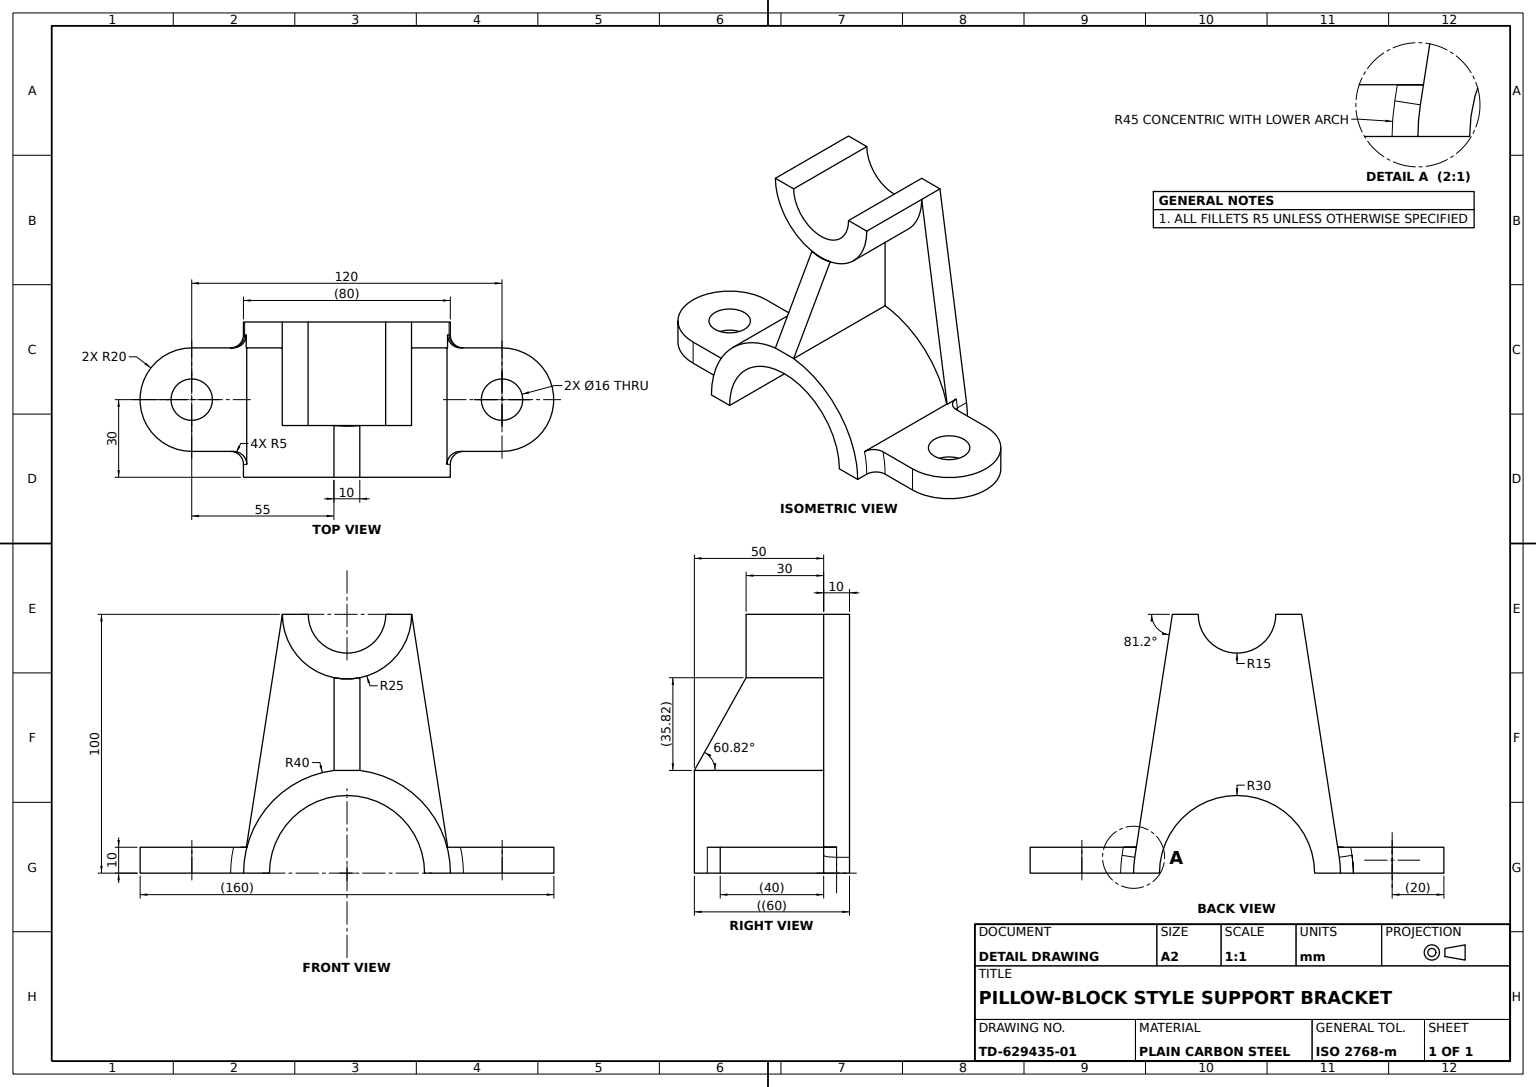
ISO-10303-21;
HEADER;
FILE_DESCRIPTION((''),'2;1');
FILE_NAME('','',(''),(''),'','','');
FILE_SCHEMA(('AUTOMOTIVE_DESIGN'));
ENDSEC;
DATA;
#1=APPLICATION_CONTEXT('');
#2=PRODUCT_CONTEXT('',#1,'mechanical');
#3=PRODUCT('','','',(#2));
#4=PRODUCT_DEFINITION_FORMATION('','',#3);
#5=PRODUCT_DEFINITION_CONTEXT('',#1,'design');
#6=PRODUCT_DEFINITION('','',#4,#5);
#7=PRODUCT_DEFINITION_SHAPE('','',#6);
#8=(LENGTH_UNIT()NAMED_UNIT(*)SI_UNIT(.MILLI.,.METRE.));
#9=(NAMED_UNIT(*)PLANE_ANGLE_UNIT()SI_UNIT($,.RADIAN.));
#10=(NAMED_UNIT(*)SI_UNIT($,.STERADIAN.)SOLID_ANGLE_UNIT());
#11=UNCERTAINTY_MEASURE_WITH_UNIT(LENGTH_MEASURE(1.E-05),#8,'distance_accuracy_value','');
#12=(GEOMETRIC_REPRESENTATION_CONTEXT(3)GLOBAL_UNCERTAINTY_ASSIGNED_CONTEXT((#11))GLOBAL_UNIT_ASSIGNED_CONTEXT((#8,#9,#10))REPRESENTATION_CONTEXT('',''));
#13=CARTESIAN_POINT('',(60.,0.,10.));
#14=VERTEX_POINT('',#13);
#15=CARTESIAN_POINT('',(60.,0.,50.));
#16=VERTEX_POINT('',#15);
#17=CARTESIAN_POINT('',(60.,0.,30.));
#18=DIRECTION('',(0.,-1.,0.));
#19=DIRECTION('',(0.,0.,-1.));
#20=AXIS2_PLACEMENT_3D('',#17,#18,#19);
#21=CIRCLE('',#20,20.);
#22=EDGE_CURVE('',#14,#16,#21,.T.);
#23=ORIENTED_EDGE('',*,*,#22,.T.);
#24=CARTESIAN_POINT('',(45.,0.,50.));
#25=VERTEX_POINT('',#24);
#26=DIRECTION('',(-1.,0.,0.));
#27=VECTOR('',#26,1000.);
#28=LINE('',#15,#27);
#29=EDGE_CURVE('',#16,#25,#28,.T.);
#30=ORIENTED_EDGE('',*,*,#29,.T.);
#31=CARTESIAN_POINT('',(40.,0.,55.));
#32=VERTEX_POINT('',#31);
#33=CARTESIAN_POINT('',(45.,0.,55.));
#34=DIRECTION('',(0.,1.,0.));
#35=DIRECTION('',(0.,0.,1.));
#36=AXIS2_PLACEMENT_3D('',#33,#34,#35);
#37=CIRCLE('',#36,5.);
#38=EDGE_CURVE('',#25,#32,#37,.T.);
#39=ORIENTED_EDGE('',*,*,#38,.T.);
#40=CARTESIAN_POINT('',(40.,0.,60.));
#41=VERTEX_POINT('',#40);
#42=CARTESIAN_POINT('',(40.,0.,50.));
#43=VECTOR('',#19,1000.);
#44=LINE('',#42,#43);
#45=EDGE_CURVE('',#41,#32,#44,.T.);
#46=ORIENTED_EDGE('',*,*,#45,.F.);
#47=CARTESIAN_POINT('',(30.,0.,60.));
#48=VERTEX_POINT('',#47);
#49=DIRECTION('',(1.,0.,0.));
#50=VECTOR('',#49,1000.);
#51=LINE('',#47,#50);
#52=EDGE_CURVE('',#48,#41,#51,.T.);
#53=ORIENTED_EDGE('',*,*,#52,.F.);
#54=CARTESIAN_POINT('',(30.,0.,0.));
#55=VERTEX_POINT('',#54);
#56=CARTESIAN_POINT('',(30.,0.,50.));
#57=LINE('',#56,#43);
#58=EDGE_CURVE('',#48,#55,#57,.T.);
#59=ORIENTED_EDGE('',*,*,#58,.T.);
#60=CARTESIAN_POINT('',(40.,0.,0.));
#61=VERTEX_POINT('',#60);
#62=LINE('',#54,#50);
#63=EDGE_CURVE('',#55,#61,#62,.T.);
#64=ORIENTED_EDGE('',*,*,#63,.T.);
#65=CARTESIAN_POINT('',(40.,0.,5.));
#66=VERTEX_POINT('',#65);
#67=EDGE_CURVE('',#66,#61,#44,.T.);
#68=ORIENTED_EDGE('',*,*,#67,.F.);
#69=CARTESIAN_POINT('',(45.,0.,10.));
#70=VERTEX_POINT('',#69);
#71=CARTESIAN_POINT('',(45.,0.,5.));
#72=AXIS2_PLACEMENT_3D('',#71,#34,#35);
#73=CIRCLE('',#72,5.);
#74=EDGE_CURVE('',#66,#70,#73,.T.);
#75=ORIENTED_EDGE('',*,*,#74,.T.);
#76=LINE('',#13,#50);
#77=EDGE_CURVE('',#70,#14,#76,.T.);
#78=ORIENTED_EDGE('',*,*,#77,.T.);
#79=EDGE_LOOP('',(#23,#30,#39,#46,#53,#59,#64,#68,#75,#78));
#80=FACE_OUTER_BOUND('',#79,.T.);
#81=CARTESIAN_POINT('',(60.,0.,22.));
#82=VERTEX_POINT('',#81);
#83=CARTESIAN_POINT('',(60.,0.,38.));
#84=VERTEX_POINT('',#83);
#85=CIRCLE('',#20,8.);
#86=EDGE_CURVE('',#82,#84,#85,.T.);
#87=ORIENTED_EDGE('',*,*,#86,.F.);
#88=EDGE_CURVE('',#84,#82,#85,.T.);
#89=ORIENTED_EDGE('',*,*,#88,.F.);
#90=EDGE_LOOP('',(#87,#89));
#91=FACE_BOUND('',#90,.T.);
#92=AXIS2_PLACEMENT_3D('',#56,#34,#35);
#93=PLANE('',#92);
#94=ADVANCED_FACE('',(#80,#91),#93,.F.);
#95=CARTESIAN_POINT('',(5.,75.505103,20.));
#96=VERTEX_POINT('',#95);
#97=CARTESIAN_POINT('',(-5.,75.505103,20.));
#98=VERTEX_POINT('',#97);
#99=CARTESIAN_POINT('',(1.689422,74.829334,19.622674));
#100=CARTESIAN_POINT('',(-1.689422,74.829334,19.622674));
#101=(BOUNDED_CURVE()B_SPLINE_CURVE(3,(#95,#99,#100,#97),.UNSPECIFIED.,.F.,.F.)B_SPLINE_CURVE_WITH_KNOTS((4,4),(2.940234733,3.342950574),.UNSPECIFIED.)CURVE()GEOMETRIC_REPRESENTATION_ITEM()RATIONAL_B_SPLINE_CURVE((1.,0.986530598,0.986530598,1.))REPRESENTATION_ITEM(''));
#102=EDGE_CURVE('',#96,#98,#101,.T.);
#103=ORIENTED_EDGE('',*,*,#102,.F.);
#104=CARTESIAN_POINT('',(5.,39.68627,0.));
#105=VERTEX_POINT('',#104);
#106=CARTESIAN_POINT('',(5.,51.162369,6.407858));
#107=DIRECTION('',(0.,0.873113733,0.487516573));
#108=VECTOR('',#107,1000.);
#109=LINE('',#106,#108);
#110=EDGE_CURVE('',#105,#96,#109,.T.);
#111=ORIENTED_EDGE('',*,*,#110,.F.);
#112=CARTESIAN_POINT('',(-5.,39.68627,0.));
#113=VERTEX_POINT('',#112);
#114=CARTESIAN_POINT('',(10.,39.68627,0.));
#115=LINE('',#114,#27);
#116=EDGE_CURVE('',#105,#113,#115,.T.);
#117=ORIENTED_EDGE('',*,*,#116,.T.);
#118=LINE('',#97,#108);
#119=EDGE_CURVE('',#113,#98,#118,.T.);
#120=ORIENTED_EDGE('',*,*,#119,.T.);
#121=EDGE_LOOP('',(#103,#111,#117,#120));
#122=FACE_OUTER_BOUND('',#121,.T.);
#123=CARTESIAN_POINT('',(10.,75.505103,20.));
#124=DIRECTION('',(0.,-0.487516573,0.873113733));
#125=DIRECTION('',(0.,-0.873113733,-0.487516573));
#126=AXIS2_PLACEMENT_3D('',#123,#124,#125);
#127=PLANE('',#126);
#128=ADVANCED_FACE('',(#122),#127,.F.);
#129=CARTESIAN_POINT('',(5.,39.68627,50.));
#130=VERTEX_POINT('',#129);
#131=CARTESIAN_POINT('',(38.729833,10.,50.));
#132=VERTEX_POINT('',#131);
#133=CARTESIAN_POINT('',(0.,0.,50.));
#134=AXIS2_PLACEMENT_3D('',#133,#19,#49);
#135=CIRCLE('',#134,40.);
#136=EDGE_CURVE('',#130,#132,#135,.T.);
#137=ORIENTED_EDGE('',*,*,#136,.T.);
#138=CARTESIAN_POINT('',(38.729833,10.,5.));
#139=VERTEX_POINT('',#138);
#140=VECTOR('',#35,1000.);
#141=LINE('',#131,#140);
#142=EDGE_CURVE('',#139,#132,#141,.T.);
#143=ORIENTED_EDGE('',*,*,#142,.F.);
#144=CARTESIAN_POINT('',(0.,0.,5.));
#145=AXIS2_PLACEMENT_3D('',#144,#19,#49);
#146=CIRCLE('',#145,40.);
#147=EDGE_CURVE('',#139,#66,#146,.T.);
#148=ORIENTED_EDGE('',*,*,#147,.T.);
#149=ORIENTED_EDGE('',*,*,#67,.T.);
#150=CARTESIAN_POINT('',(0.,0.,0.));
#151=AXIS2_PLACEMENT_3D('',#150,#35,#49);
#152=CIRCLE('',#151,40.);
#153=EDGE_CURVE('',#61,#105,#152,.T.);
#154=ORIENTED_EDGE('',*,*,#153,.T.);
#155=CARTESIAN_POINT('',(5.,39.68627,-37.188557));
#156=LINE('',#155,#140);
#157=EDGE_CURVE('',#105,#130,#156,.T.);
#158=ORIENTED_EDGE('',*,*,#157,.T.);
#159=EDGE_LOOP('',(#137,#143,#148,#149,#154,#158));
#160=FACE_OUTER_BOUND('',#159,.T.);
#161=AXIS2_PLACEMENT_3D('',#133,#19,#26);
#162=CYLINDRICAL_SURFACE('',#161,40.);
#163=ADVANCED_FACE('',(#160),#162,.T.);
#164=ORIENTED_EDGE('',*,*,#77,.F.);
#165=CARTESIAN_POINT('',(43.874822,10.,10.));
#166=VERTEX_POINT('',#165);
#167=CARTESIAN_POINT('',(0.,0.,10.));
#168=AXIS2_PLACEMENT_3D('',#167,#35,#49);
#169=CIRCLE('',#168,45.);
#170=EDGE_CURVE('',#70,#166,#169,.T.);
#171=ORIENTED_EDGE('',*,*,#170,.T.);
#172=CARTESIAN_POINT('',(60.,10.,10.));
#173=VERTEX_POINT('',#172);
#174=CARTESIAN_POINT('',(35.,10.,10.));
#175=LINE('',#174,#50);
#176=EDGE_CURVE('',#166,#173,#175,.T.);
#177=ORIENTED_EDGE('',*,*,#176,.T.);
#178=VECTOR('',#18,1000.);
#179=LINE('',#172,#178);
#180=EDGE_CURVE('',#173,#14,#179,.T.);
#181=ORIENTED_EDGE('',*,*,#180,.T.);
#182=EDGE_LOOP('',(#164,#171,#177,#181));
#183=FACE_OUTER_BOUND('',#182,.T.);
#184=AXIS2_PLACEMENT_3D('',#174,#35,#49);
#185=PLANE('',#184);
#186=ADVANCED_FACE('',(#183),#185,.F.);
#187=ORIENTED_EDGE('',*,*,#157,.F.);
#188=ORIENTED_EDGE('',*,*,#110,.T.);
#189=CARTESIAN_POINT('',(5.,75.505103,50.));
#190=VERTEX_POINT('',#189);
#191=CARTESIAN_POINT('',(5.,75.505103,-37.188557));
#192=LINE('',#191,#140);
#193=EDGE_CURVE('',#96,#190,#192,.T.);
#194=ORIENTED_EDGE('',*,*,#193,.T.);
#195=LINE('',#189,#178);
#196=EDGE_CURVE('',#190,#130,#195,.T.);
#197=ORIENTED_EDGE('',*,*,#196,.T.);
#198=EDGE_LOOP('',(#187,#188,#194,#197));
#199=FACE_OUTER_BOUND('',#198,.T.);
#200=AXIS2_PLACEMENT_3D('',#191,#26,#35);
#201=PLANE('',#200);
#202=ADVANCED_FACE('',(#199),#201,.F.);
#203=CARTESIAN_POINT('',(-43.874822,10.,10.));
#204=VERTEX_POINT('',#203);
#205=CARTESIAN_POINT('',(-45.,0.,10.));
#206=VERTEX_POINT('',#205);
#207=EDGE_CURVE('',#204,#206,#169,.T.);
#208=ORIENTED_EDGE('',*,*,#207,.F.);
#209=CARTESIAN_POINT('',(-38.729833,10.,5.));
#210=VERTEX_POINT('',#209);
#211=CARTESIAN_POINT('',(-38.729833,10.,5.334921));
#212=CARTESIAN_POINT('',(-38.764239,10.,5.663939));
#213=CARTESIAN_POINT('',(-38.898767,10.,6.310699));
#214=CARTESIAN_POINT('',(-39.000686,10.,6.631925));
#215=CARTESIAN_POINT('',(-39.26464,10.,7.240754));
#216=CARTESIAN_POINT('',(-39.425819,10.,7.528988));
#217=CARTESIAN_POINT('',(-39.805716,10.,8.073571));
#218=CARTESIAN_POINT('',(-40.024896,10.,8.328981));
#219=CARTESIAN_POINT('',(-40.501992,10.,8.786245));
#220=CARTESIAN_POINT('',(-40.762043,10.,8.99135));
#221=CARTESIAN_POINT('',(-41.325287,10.,9.352802));
#222=CARTESIAN_POINT('',(-41.619798,10.,9.503625));
#223=CARTESIAN_POINT('',(-42.233333,10.,9.748401));
#224=CARTESIAN_POINT('',(-42.555336,10.,9.842795));
#225=CARTESIAN_POINT('',(-43.209353,10.,9.968362));
#226=CARTESIAN_POINT('',(-43.540159,10.,10.));
#227=B_SPLINE_CURVE_WITH_KNOTS('',3,(#209,#211,#212,#213,#214,#215,#216,#217,#218,#219,#220,#221,#222,#223,#224,#225,#226,#203),.UNSPECIFIED.,.F.,.F.,(4,2,2,2,2,2,2,2,4),(0.,0.000990292,0.001980584,0.002970876,0.003961168,0.00495146,0.005941752,0.006932044,0.007922336),.UNSPECIFIED.);
#228=EDGE_CURVE('',#210,#204,#227,.T.);
#229=ORIENTED_EDGE('',*,*,#228,.F.);
#230=CARTESIAN_POINT('',(-40.,0.,5.));
#231=VERTEX_POINT('',#230);
#232=EDGE_CURVE('',#231,#210,#146,.T.);
#233=ORIENTED_EDGE('',*,*,#232,.F.);
#234=CARTESIAN_POINT('',(-45.,0.,5.));
#235=AXIS2_PLACEMENT_3D('',#234,#34,#35);
#236=CIRCLE('',#235,5.);
#237=EDGE_CURVE('',#206,#231,#236,.T.);
#238=ORIENTED_EDGE('',*,*,#237,.F.);
#239=EDGE_LOOP('',(#208,#229,#233,#238));
#240=FACE_OUTER_BOUND('',#239,.T.);
#241=AXIS2_PLACEMENT_3D('',#144,#35,#49);
#242=TOROIDAL_SURFACE('',#241,45.,5.);
#243=ADVANCED_FACE('',(#240),#242,.F.);
#244=ORIENTED_EDGE('',*,*,#147,.F.);
#245=CARTESIAN_POINT('',(43.539992,10.,10.));
#246=CARTESIAN_POINT('',(43.21054,10.,9.968335));
#247=CARTESIAN_POINT('',(42.724094,10.,9.875321));
#248=CARTESIAN_POINT('',(42.563243,10.,9.836674));
#249=CARTESIAN_POINT('',(42.244192,10.,9.743772));
#250=CARTESIAN_POINT('',(42.085245,10.,9.689167));
#251=CARTESIAN_POINT('',(41.621523,10.,9.504613));
#252=CARTESIAN_POINT('',(41.327745,10.,9.353874));
#253=CARTESIAN_POINT('',(40.770701,10.,8.997402));
#254=CARTESIAN_POINT('',(40.505176,10.,8.788985));
#255=CARTESIAN_POINT('',(40.026677,10.,8.330996));
#256=CARTESIAN_POINT('',(39.811545,10.,8.080827));
#257=CARTESIAN_POINT('',(39.525925,10.,7.673018));
#258=CARTESIAN_POINT('',(39.436488,10.,7.530735));
#259=CARTESIAN_POINT('',(39.273687,10.,7.240064));
#260=CARTESIAN_POINT('',(39.200154,10.,7.091651));
#261=CARTESIAN_POINT('',(39.002728,10.,6.637342));
#262=CARTESIAN_POINT('',(38.901772,10.,6.322474));
#263=CARTESIAN_POINT('',(38.764431,10.,5.667473));
#264=CARTESIAN_POINT('',(38.729833,10.,5.335102));
#265=B_SPLINE_CURVE_WITH_KNOTS('',3,(#165,#245,#246,#247,#248,#249,#250,#251,#252,#253,#254,#255,#256,#257,#258,#259,#260,#261,#262,#263,#264,#138),.UNSPECIFIED.,.F.,.F.,(4,2,2,2,2,2,2,2,2,2,4),(0.,0.000990307,0.001485461,0.001980615,0.002970922,0.003961229,0.004951537,0.00544669,0.005941844,0.006932151,0.007922459),.UNSPECIFIED.);
#266=EDGE_CURVE('',#166,#139,#265,.T.);
#267=ORIENTED_EDGE('',*,*,#266,.F.);
#268=ORIENTED_EDGE('',*,*,#170,.F.);
#269=ORIENTED_EDGE('',*,*,#74,.F.);
#270=EDGE_LOOP('',(#244,#267,#268,#269));
#271=FACE_OUTER_BOUND('',#270,.T.);
#272=ADVANCED_FACE('',(#271),#242,.F.);
#273=CARTESIAN_POINT('',(44.470588,6.882353,50.));
#274=VERTEX_POINT('',#273);
#275=CIRCLE('',#161,45.);
#276=EDGE_CURVE('',#274,#25,#275,.T.);
#277=ORIENTED_EDGE('',*,*,#276,.F.);
#278=CARTESIAN_POINT('',(39.529412,6.117647,55.));
#279=VERTEX_POINT('',#278);
#280=CARTESIAN_POINT('',(44.470588,6.882353,55.));
#281=DIRECTION('',(0.152941176,-0.988235294,0.));
#282=DIRECTION('',(0.988235294,0.152941176,0.));
#283=AXIS2_PLACEMENT_3D('',#280,#281,#282);
#284=CIRCLE('',#283,5.);
#285=EDGE_CURVE('',#279,#274,#284,.T.);
#286=ORIENTED_EDGE('',*,*,#285,.F.);
#287=CARTESIAN_POINT('',(0.,0.,55.));
#288=AXIS2_PLACEMENT_3D('',#287,#35,#26);
#289=CIRCLE('',#288,40.);
#290=EDGE_CURVE('',#32,#279,#289,.T.);
#291=ORIENTED_EDGE('',*,*,#290,.F.);
#292=ORIENTED_EDGE('',*,*,#38,.F.);
#293=EDGE_LOOP('',(#277,#286,#291,#292));
#294=FACE_OUTER_BOUND('',#293,.T.);
#295=AXIS2_PLACEMENT_3D('',#287,#19,#26);
#296=TOROIDAL_SURFACE('',#295,45.,5.);
#297=ADVANCED_FACE('',(#294),#296,.F.);
#298=CARTESIAN_POINT('',(60.,10.,38.));
#299=VERTEX_POINT('',#298);
#300=CARTESIAN_POINT('',(60.,10.,22.));
#301=VERTEX_POINT('',#300);
#302=CARTESIAN_POINT('',(60.,10.,30.));
#303=AXIS2_PLACEMENT_3D('',#302,#18,#19);
#304=CIRCLE('',#303,8.);
#305=EDGE_CURVE('',#299,#301,#304,.T.);
#306=ORIENTED_EDGE('',*,*,#305,.T.);
#307=EDGE_CURVE('',#301,#299,#304,.T.);
#308=ORIENTED_EDGE('',*,*,#307,.T.);
#309=EDGE_LOOP('',(#306,#308));
#310=FACE_BOUND('',#309,.T.);
#311=ORIENTED_EDGE('',*,*,#266,.T.);
#312=ORIENTED_EDGE('',*,*,#142,.T.);
#313=CARTESIAN_POINT('',(38.928571,10.,50.));
#314=VERTEX_POINT('',#313);
#315=CARTESIAN_POINT('',(35.,10.,50.));
#316=LINE('',#315,#50);
#317=EDGE_CURVE('',#132,#314,#316,.T.);
#318=ORIENTED_EDGE('',*,*,#317,.T.);
#319=CARTESIAN_POINT('',(38.928571,10.,55.));
#320=VERTEX_POINT('',#319);
#321=LINE('',#313,#43);
#322=EDGE_CURVE('',#320,#314,#321,.T.);
#323=ORIENTED_EDGE('',*,*,#322,.F.);
#324=CARTESIAN_POINT('',(43.988095,10.,50.));
#325=VERTEX_POINT('',#324);
#326=CARTESIAN_POINT('',(38.928571,10.,52.071068));
#327=CARTESIAN_POINT('',(41.024295,10.,50.));
#328=(BOUNDED_CURVE()B_SPLINE_CURVE(3,(#319,#326,#327,#324),.UNSPECIFIED.,.F.,.F.)B_SPLINE_CURVE_WITH_KNOTS((4,4),(3.141592654,4.71238898),.UNSPECIFIED.)CURVE()GEOMETRIC_REPRESENTATION_ITEM()RATIONAL_B_SPLINE_CURVE((1.,0.804737854,0.804737854,1.))REPRESENTATION_ITEM(''));
#329=EDGE_CURVE('',#320,#325,#328,.T.);
#330=ORIENTED_EDGE('',*,*,#329,.T.);
#331=CARTESIAN_POINT('',(60.,10.,50.));
#332=VERTEX_POINT('',#331);
#333=EDGE_CURVE('',#325,#332,#316,.T.);
#334=ORIENTED_EDGE('',*,*,#333,.T.);
#335=CIRCLE('',#303,20.);
#336=EDGE_CURVE('',#173,#332,#335,.T.);
#337=ORIENTED_EDGE('',*,*,#336,.F.);
#338=ORIENTED_EDGE('',*,*,#176,.F.);
#339=EDGE_LOOP('',(#311,#312,#318,#323,#330,#334,#337,#338));
#340=FACE_OUTER_BOUND('',#339,.T.);
#341=AXIS2_PLACEMENT_3D('',#315,#18,#19);
#342=PLANE('',#341);
#343=ADVANCED_FACE('',(#310,#340),#342,.F.);
#344=CARTESIAN_POINT('',(25.,100.,50.));
#345=VERTEX_POINT('',#344);
#346=CARTESIAN_POINT('',(0.,100.,50.));
#347=AXIS2_PLACEMENT_3D('',#346,#19,#49);
#348=CIRCLE('',#347,25.);
#349=EDGE_CURVE('',#345,#190,#348,.T.);
#350=ORIENTED_EDGE('',*,*,#349,.T.);
#351=ORIENTED_EDGE('',*,*,#193,.F.);
#352=CARTESIAN_POINT('',(25.,100.,20.));
#353=VERTEX_POINT('',#352);
#354=CARTESIAN_POINT('',(0.,100.,20.));
#355=AXIS2_PLACEMENT_3D('',#354,#35,#49);
#356=CIRCLE('',#355,25.);
#357=EDGE_CURVE('',#96,#353,#356,.T.);
#358=ORIENTED_EDGE('',*,*,#357,.T.);
#359=LINE('',#352,#140);
#360=EDGE_CURVE('',#353,#345,#359,.T.);
#361=ORIENTED_EDGE('',*,*,#360,.T.);
#362=EDGE_LOOP('',(#350,#351,#358,#361));
#363=FACE_OUTER_BOUND('',#362,.T.);
#364=CYLINDRICAL_SURFACE('',#355,25.);
#365=ADVANCED_FACE('',(#363),#364,.T.);
#366=ORIENTED_EDGE('',*,*,#307,.F.);
#367=LINE('',#300,#178);
#368=EDGE_CURVE('',#301,#82,#367,.T.);
#369=ORIENTED_EDGE('',*,*,#368,.T.);
#370=ORIENTED_EDGE('',*,*,#86,.T.);
#371=LINE('',#298,#178);
#372=EDGE_CURVE('',#299,#84,#371,.T.);
#373=ORIENTED_EDGE('',*,*,#372,.F.);
#374=EDGE_LOOP('',(#366,#369,#370,#373));
#375=FACE_OUTER_BOUND('',#374,.T.);
#376=CYLINDRICAL_SURFACE('',#303,8.);
#377=ADVANCED_FACE('',(#375),#376,.F.);
#378=ORIENTED_EDGE('',*,*,#317,.F.);
#379=ORIENTED_EDGE('',*,*,#136,.F.);
#380=ORIENTED_EDGE('',*,*,#196,.F.);
#381=ORIENTED_EDGE('',*,*,#349,.F.);
#382=DIRECTION('',(-0.152941176,0.988235294,0.));
#383=VECTOR('',#382,1000.);
#384=LINE('',#344,#383);
#385=EDGE_CURVE('',#314,#345,#384,.T.);
#386=ORIENTED_EDGE('',*,*,#385,.F.);
#387=EDGE_LOOP('',(#378,#379,#380,#381,#386));
#388=FACE_OUTER_BOUND('',#387,.T.);
#389=AXIS2_PLACEMENT_3D('',#346,#35,#49);
#390=PLANE('',#389);
#391=ADVANCED_FACE('',(#388),#390,.F.);
#392=CARTESIAN_POINT('',(-25.,100.,20.));
#393=VERTEX_POINT('',#392);
#394=EDGE_CURVE('',#393,#98,#356,.T.);
#395=ORIENTED_EDGE('',*,*,#394,.F.);
#396=CARTESIAN_POINT('',(-15.,100.,20.));
#397=VERTEX_POINT('',#396);
#398=LINE('',#392,#27);
#399=EDGE_CURVE('',#397,#393,#398,.T.);
#400=ORIENTED_EDGE('',*,*,#399,.F.);
#401=CARTESIAN_POINT('',(15.,100.,20.));
#402=VERTEX_POINT('',#401);
#403=AXIS2_PLACEMENT_3D('',#354,#19,#49);
#404=CIRCLE('',#403,15.);
#405=EDGE_CURVE('',#402,#397,#404,.T.);
#406=ORIENTED_EDGE('',*,*,#405,.F.);
#407=LINE('',#401,#27);
#408=EDGE_CURVE('',#353,#402,#407,.T.);
#409=ORIENTED_EDGE('',*,*,#408,.F.);
#410=ORIENTED_EDGE('',*,*,#357,.F.);
#411=EDGE_CURVE('',#98,#96,#356,.T.);
#412=ORIENTED_EDGE('',*,*,#411,.F.);
#413=EDGE_LOOP('',(#395,#400,#406,#409,#410,#412));
#414=FACE_OUTER_BOUND('',#413,.T.);
#415=PLANE('',#355);
#416=ADVANCED_FACE('',(#414),#415,.F.);
#417=ORIENTED_EDGE('',*,*,#411,.T.);
#418=ORIENTED_EDGE('',*,*,#102,.T.);
#419=EDGE_LOOP('',(#417,#418));
#420=FACE_OUTER_BOUND('',#419,.T.);
#421=CARTESIAN_POINT('',(0.,100.,-37.188557));
#422=AXIS2_PLACEMENT_3D('',#421,#35,#49);
#423=CYLINDRICAL_SURFACE('',#422,25.);
#424=ADVANCED_FACE('',(#420),#423,.F.);
#425=CARTESIAN_POINT('',(-60.,0.,38.));
#426=VERTEX_POINT('',#425);
#427=CARTESIAN_POINT('',(-60.,0.,22.));
#428=VERTEX_POINT('',#427);
#429=CARTESIAN_POINT('',(-60.,0.,30.));
#430=AXIS2_PLACEMENT_3D('',#429,#18,#19);
#431=CIRCLE('',#430,8.);
#432=EDGE_CURVE('',#426,#428,#431,.T.);
#433=ORIENTED_EDGE('',*,*,#432,.T.);
#434=CARTESIAN_POINT('',(-60.,10.,22.));
#435=VERTEX_POINT('',#434);
#436=LINE('',#434,#178);
#437=EDGE_CURVE('',#435,#428,#436,.T.);
#438=ORIENTED_EDGE('',*,*,#437,.F.);
#439=CARTESIAN_POINT('',(-60.,10.,38.));
#440=VERTEX_POINT('',#439);
#441=CARTESIAN_POINT('',(-60.,10.,30.));
#442=AXIS2_PLACEMENT_3D('',#441,#18,#19);
#443=CIRCLE('',#442,8.);
#444=EDGE_CURVE('',#440,#435,#443,.T.);
#445=ORIENTED_EDGE('',*,*,#444,.F.);
#446=LINE('',#439,#178);
#447=EDGE_CURVE('',#440,#426,#446,.T.);
#448=ORIENTED_EDGE('',*,*,#447,.T.);
#449=EDGE_LOOP('',(#433,#438,#445,#448));
#450=FACE_OUTER_BOUND('',#449,.T.);
#451=CYLINDRICAL_SURFACE('',#442,8.);
#452=ADVANCED_FACE('',(#450),#451,.F.);
#453=ORIENTED_EDGE('',*,*,#372,.T.);
#454=ORIENTED_EDGE('',*,*,#88,.T.);
#455=ORIENTED_EDGE('',*,*,#368,.F.);
#456=ORIENTED_EDGE('',*,*,#305,.F.);
#457=EDGE_LOOP('',(#453,#454,#455,#456));
#458=FACE_OUTER_BOUND('',#457,.T.);
#459=ADVANCED_FACE('',(#458),#376,.F.);
#460=ORIENTED_EDGE('',*,*,#276,.T.);
#461=ORIENTED_EDGE('',*,*,#29,.F.);
#462=LINE('',#331,#178);
#463=EDGE_CURVE('',#332,#16,#462,.T.);
#464=ORIENTED_EDGE('',*,*,#463,.F.);
#465=ORIENTED_EDGE('',*,*,#333,.F.);
#466=VECTOR('',#281,1000.);
#467=LINE('',#273,#466);
#468=EDGE_CURVE('',#325,#274,#467,.T.);
#469=ORIENTED_EDGE('',*,*,#468,.T.);
#470=EDGE_LOOP('',(#460,#461,#464,#465,#469));
#471=FACE_OUTER_BOUND('',#470,.T.);
#472=CARTESIAN_POINT('',(35.,0.,50.));
#473=AXIS2_PLACEMENT_3D('',#472,#19,#26);
#474=PLANE('',#473);
#475=ADVANCED_FACE('',(#471),#474,.F.);
#476=CARTESIAN_POINT('',(-15.,100.,60.));
#477=VERTEX_POINT('',#476);
#478=CARTESIAN_POINT('',(-25.,100.,60.));
#479=VERTEX_POINT('',#478);
#480=LINE('',#476,#27);
#481=EDGE_CURVE('',#477,#479,#480,.T.);
#482=ORIENTED_EDGE('',*,*,#481,.F.);
#483=LINE('',#396,#140);
#484=EDGE_CURVE('',#397,#477,#483,.T.);
#485=ORIENTED_EDGE('',*,*,#484,.F.);
#486=ORIENTED_EDGE('',*,*,#399,.T.);
#487=CARTESIAN_POINT('',(-25.,100.,50.));
#488=VERTEX_POINT('',#487);
#489=LINE('',#392,#140);
#490=EDGE_CURVE('',#393,#488,#489,.T.);
#491=ORIENTED_EDGE('',*,*,#490,.T.);
#492=LINE('',#478,#43);
#493=EDGE_CURVE('',#479,#488,#492,.T.);
#494=ORIENTED_EDGE('',*,*,#493,.F.);
#495=EDGE_LOOP('',(#482,#485,#486,#491,#494));
#496=FACE_OUTER_BOUND('',#495,.T.);
#497=AXIS2_PLACEMENT_3D('',#392,#34,#35);
#498=PLANE('',#497);
#499=ADVANCED_FACE('',(#496),#498,.T.);
#500=ORIENTED_EDGE('',*,*,#437,.T.);
#501=EDGE_CURVE('',#428,#426,#431,.T.);
#502=ORIENTED_EDGE('',*,*,#501,.T.);
#503=ORIENTED_EDGE('',*,*,#447,.F.);
#504=EDGE_CURVE('',#435,#440,#443,.T.);
#505=ORIENTED_EDGE('',*,*,#504,.F.);
#506=EDGE_LOOP('',(#500,#502,#503,#505));
#507=FACE_OUTER_BOUND('',#506,.T.);
#508=ADVANCED_FACE('',(#507),#451,.F.);
#509=CARTESIAN_POINT('',(-60.,10.,10.));
#510=VERTEX_POINT('',#509);
#511=CARTESIAN_POINT('',(-35.,10.,10.));
#512=LINE('',#511,#27);
#513=EDGE_CURVE('',#204,#510,#512,.T.);
#514=ORIENTED_EDGE('',*,*,#513,.F.);
#515=ORIENTED_EDGE('',*,*,#207,.T.);
#516=CARTESIAN_POINT('',(-60.,0.,10.));
#517=VERTEX_POINT('',#516);
#518=LINE('',#516,#50);
#519=EDGE_CURVE('',#517,#206,#518,.T.);
#520=ORIENTED_EDGE('',*,*,#519,.F.);
#521=LINE('',#509,#178);
#522=EDGE_CURVE('',#510,#517,#521,.T.);
#523=ORIENTED_EDGE('',*,*,#522,.F.);
#524=EDGE_LOOP('',(#514,#515,#520,#523));
#525=FACE_OUTER_BOUND('',#524,.T.);
#526=CARTESIAN_POINT('',(-35.,0.,10.));
#527=AXIS2_PLACEMENT_3D('',#526,#35,#49);
#528=PLANE('',#527);
#529=ADVANCED_FACE('',(#525),#528,.F.);
#530=ORIENTED_EDGE('',*,*,#493,.T.);
#531=CARTESIAN_POINT('',(-38.928571,10.,50.));
#532=VERTEX_POINT('',#531);
#533=DIRECTION('',(-0.152941176,-0.988235294,0.));
#534=VECTOR('',#533,1000.);
#535=LINE('',#487,#534);
#536=EDGE_CURVE('',#488,#532,#535,.T.);
#537=ORIENTED_EDGE('',*,*,#536,.T.);
#538=CARTESIAN_POINT('',(-38.928571,10.,55.));
#539=VERTEX_POINT('',#538);
#540=CARTESIAN_POINT('',(-38.928571,10.,10.));
#541=LINE('',#540,#140);
#542=EDGE_CURVE('',#532,#539,#541,.T.);
#543=ORIENTED_EDGE('',*,*,#542,.T.);
#544=CARTESIAN_POINT('',(-39.529412,6.117647,55.));
#545=VERTEX_POINT('',#544);
#546=LINE('',#544,#534);
#547=EDGE_CURVE('',#539,#545,#546,.T.);
#548=ORIENTED_EDGE('',*,*,#547,.T.);
#549=CARTESIAN_POINT('',(-39.529412,6.117647,60.));
#550=VERTEX_POINT('',#549);
#551=LINE('',#549,#43);
#552=EDGE_CURVE('',#550,#545,#551,.T.);
#553=ORIENTED_EDGE('',*,*,#552,.F.);
#554=LINE('',#478,#534);
#555=EDGE_CURVE('',#479,#550,#554,.T.);
#556=ORIENTED_EDGE('',*,*,#555,.F.);
#557=EDGE_LOOP('',(#530,#537,#543,#548,#553,#556));
#558=FACE_OUTER_BOUND('',#557,.T.);
#559=DIRECTION('',(0.988235294,-0.152941176,0.));
#560=DIRECTION('',(0.152941176,0.988235294,0.));
#561=AXIS2_PLACEMENT_3D('',#478,#559,#560);
#562=PLANE('',#561);
#563=ADVANCED_FACE('',(#558),#562,.F.);
#564=CARTESIAN_POINT('',(-40.,0.,0.));
#565=VERTEX_POINT('',#564);
#566=EDGE_CURVE('',#113,#565,#152,.T.);
#567=ORIENTED_EDGE('',*,*,#566,.F.);
#568=ORIENTED_EDGE('',*,*,#116,.F.);
#569=ORIENTED_EDGE('',*,*,#153,.F.);
#570=ORIENTED_EDGE('',*,*,#63,.F.);
#571=CARTESIAN_POINT('',(-30.,0.,0.));
#572=VERTEX_POINT('',#571);
#573=AXIS2_PLACEMENT_3D('',#150,#19,#49);
#574=CIRCLE('',#573,30.);
#575=EDGE_CURVE('',#572,#55,#574,.T.);
#576=ORIENTED_EDGE('',*,*,#575,.F.);
#577=LINE('',#564,#50);
#578=EDGE_CURVE('',#565,#572,#577,.T.);
#579=ORIENTED_EDGE('',*,*,#578,.F.);
#580=EDGE_LOOP('',(#567,#568,#569,#570,#576,#579));
#581=FACE_OUTER_BOUND('',#580,.T.);
#582=PLANE('',#151);
#583=ADVANCED_FACE('',(#581),#582,.F.);
#584=CARTESIAN_POINT('',(-60.,10.,50.));
#585=VERTEX_POINT('',#584);
#586=CIRCLE('',#442,20.);
#587=EDGE_CURVE('',#585,#510,#586,.T.);
#588=ORIENTED_EDGE('',*,*,#587,.T.);
#589=ORIENTED_EDGE('',*,*,#522,.T.);
#590=CARTESIAN_POINT('',(-60.,0.,50.));
#591=VERTEX_POINT('',#590);
#592=CIRCLE('',#430,20.);
#593=EDGE_CURVE('',#591,#517,#592,.T.);
#594=ORIENTED_EDGE('',*,*,#593,.F.);
#595=LINE('',#584,#178);
#596=EDGE_CURVE('',#585,#591,#595,.T.);
#597=ORIENTED_EDGE('',*,*,#596,.F.);
#598=EDGE_LOOP('',(#588,#589,#594,#597));
#599=FACE_OUTER_BOUND('',#598,.T.);
#600=CYLINDRICAL_SURFACE('',#442,20.);
#601=ADVANCED_FACE('',(#599),#600,.T.);
#602=ORIENTED_EDGE('',*,*,#432,.F.);
#603=ORIENTED_EDGE('',*,*,#501,.F.);
#604=EDGE_LOOP('',(#602,#603));
#605=FACE_BOUND('',#604,.T.);
#606=CARTESIAN_POINT('',(-45.,0.,50.));
#607=VERTEX_POINT('',#606);
#608=LINE('',#590,#27);
#609=EDGE_CURVE('',#607,#591,#608,.T.);
#610=ORIENTED_EDGE('',*,*,#609,.T.);
#611=ORIENTED_EDGE('',*,*,#593,.T.);
#612=ORIENTED_EDGE('',*,*,#519,.T.);
#613=ORIENTED_EDGE('',*,*,#237,.T.);
#614=CARTESIAN_POINT('',(-40.,0.,50.));
#615=LINE('',#614,#43);
#616=EDGE_CURVE('',#231,#565,#615,.T.);
#617=ORIENTED_EDGE('',*,*,#616,.T.);
#618=ORIENTED_EDGE('',*,*,#578,.T.);
#619=CARTESIAN_POINT('',(-30.,0.,60.));
#620=VERTEX_POINT('',#619);
#621=CARTESIAN_POINT('',(-30.,0.,50.));
#622=LINE('',#621,#43);
#623=EDGE_CURVE('',#620,#572,#622,.T.);
#624=ORIENTED_EDGE('',*,*,#623,.F.);
#625=CARTESIAN_POINT('',(-40.,0.,60.));
#626=VERTEX_POINT('',#625);
#627=LINE('',#625,#50);
#628=EDGE_CURVE('',#626,#620,#627,.T.);
#629=ORIENTED_EDGE('',*,*,#628,.F.);
#630=CARTESIAN_POINT('',(-40.,0.,55.));
#631=VERTEX_POINT('',#630);
#632=EDGE_CURVE('',#626,#631,#615,.T.);
#633=ORIENTED_EDGE('',*,*,#632,.T.);
#634=CARTESIAN_POINT('',(-45.,0.,55.));
#635=AXIS2_PLACEMENT_3D('',#634,#34,#35);
#636=CIRCLE('',#635,5.);
#637=EDGE_CURVE('',#631,#607,#636,.T.);
#638=ORIENTED_EDGE('',*,*,#637,.T.);
#639=EDGE_LOOP('',(#610,#611,#612,#613,#617,#618,#624,#629,#633,#638));
#640=FACE_OUTER_BOUND('',#639,.T.);
#641=AXIS2_PLACEMENT_3D('',#614,#34,#35);
#642=PLANE('',#641);
#643=ADVANCED_FACE('',(#605,#640),#642,.F.);
#644=CARTESIAN_POINT('',(-5.,75.505103,50.));
#645=VERTEX_POINT('',#644);
#646=CARTESIAN_POINT('',(-5.,75.505103,-37.188557));
#647=LINE('',#646,#140);
#648=EDGE_CURVE('',#98,#645,#647,.T.);
#649=ORIENTED_EDGE('',*,*,#648,.F.);
#650=ORIENTED_EDGE('',*,*,#119,.F.);
#651=CARTESIAN_POINT('',(-5.,39.68627,50.));
#652=VERTEX_POINT('',#651);
#653=CARTESIAN_POINT('',(-5.,39.68627,-37.188557));
#654=LINE('',#653,#140);
#655=EDGE_CURVE('',#113,#652,#654,.T.);
#656=ORIENTED_EDGE('',*,*,#655,.T.);
#657=VECTOR('',#34,1000.);
#658=LINE('',#644,#657);
#659=EDGE_CURVE('',#652,#645,#658,.T.);
#660=ORIENTED_EDGE('',*,*,#659,.T.);
#661=EDGE_LOOP('',(#649,#650,#656,#660));
#662=FACE_OUTER_BOUND('',#661,.T.);
#663=AXIS2_PLACEMENT_3D('',#646,#49,#34);
#664=PLANE('',#663);
#665=ADVANCED_FACE('',(#662),#664,.F.);
#666=CARTESIAN_POINT('',(-43.988095,10.,50.));
#667=VERTEX_POINT('',#666);
#668=CARTESIAN_POINT('',(-35.,10.,50.));
#669=LINE('',#668,#27);
#670=EDGE_CURVE('',#667,#585,#669,.T.);
#671=ORIENTED_EDGE('',*,*,#670,.T.);
#672=ORIENTED_EDGE('',*,*,#596,.T.);
#673=ORIENTED_EDGE('',*,*,#609,.F.);
#674=CARTESIAN_POINT('',(-44.470588,6.882353,50.));
#675=VERTEX_POINT('',#674);
#676=EDGE_CURVE('',#607,#675,#275,.T.);
#677=ORIENTED_EDGE('',*,*,#676,.T.);
#678=CARTESIAN_POINT('',(-43.869748,10.764706,50.));
#679=VECTOR('',#560,1000.);
#680=LINE('',#678,#679);
#681=EDGE_CURVE('',#675,#667,#680,.T.);
#682=ORIENTED_EDGE('',*,*,#681,.T.);
#683=EDGE_LOOP('',(#671,#672,#673,#677,#682));
#684=FACE_OUTER_BOUND('',#683,.T.);
#685=AXIS2_PLACEMENT_3D('',#668,#19,#26);
#686=PLANE('',#685);
#687=ADVANCED_FACE('',(#684),#686,.F.);
#688=ORIENTED_EDGE('',*,*,#575,.T.);
#689=ORIENTED_EDGE('',*,*,#58,.F.);
#690=CARTESIAN_POINT('',(0.,0.,60.));
#691=AXIS2_PLACEMENT_3D('',#690,#19,#49);
#692=CIRCLE('',#691,30.);
#693=EDGE_CURVE('',#620,#48,#692,.T.);
#694=ORIENTED_EDGE('',*,*,#693,.F.);
#695=ORIENTED_EDGE('',*,*,#623,.T.);
#696=EDGE_LOOP('',(#688,#689,#694,#695));
#697=FACE_OUTER_BOUND('',#696,.T.);
#698=CYLINDRICAL_SURFACE('',#161,30.);
#699=ADVANCED_FACE('',(#697),#698,.F.);
#700=LINE('',#319,#383);
#701=EDGE_CURVE('',#279,#320,#700,.T.);
#702=ORIENTED_EDGE('',*,*,#701,.T.);
#703=ORIENTED_EDGE('',*,*,#322,.T.);
#704=ORIENTED_EDGE('',*,*,#385,.T.);
#705=CARTESIAN_POINT('',(25.,100.,60.));
#706=VERTEX_POINT('',#705);
#707=LINE('',#705,#43);
#708=EDGE_CURVE('',#706,#345,#707,.T.);
#709=ORIENTED_EDGE('',*,*,#708,.F.);
#710=CARTESIAN_POINT('',(39.529412,6.117647,60.));
#711=VERTEX_POINT('',#710);
#712=LINE('',#705,#383);
#713=EDGE_CURVE('',#711,#706,#712,.T.);
#714=ORIENTED_EDGE('',*,*,#713,.F.);
#715=LINE('',#710,#43);
#716=EDGE_CURVE('',#711,#279,#715,.T.);
#717=ORIENTED_EDGE('',*,*,#716,.T.);
#718=EDGE_LOOP('',(#702,#703,#704,#709,#714,#717));
#719=FACE_OUTER_BOUND('',#718,.T.);
#720=DIRECTION('',(-0.988235294,-0.152941176,0.));
#721=AXIS2_PLACEMENT_3D('',#705,#720,#281);
#722=PLANE('',#721);
#723=ADVANCED_FACE('',(#719),#722,.F.);
#724=ORIENTED_EDGE('',*,*,#394,.T.);
#725=ORIENTED_EDGE('',*,*,#648,.T.);
#726=EDGE_CURVE('',#645,#488,#348,.T.);
#727=ORIENTED_EDGE('',*,*,#726,.T.);
#728=ORIENTED_EDGE('',*,*,#490,.F.);
#729=EDGE_LOOP('',(#724,#725,#727,#728));
#730=FACE_OUTER_BOUND('',#729,.T.);
#731=ADVANCED_FACE('',(#730),#364,.T.);
#732=ORIENTED_EDGE('',*,*,#484,.T.);
#733=CARTESIAN_POINT('',(15.,100.,60.));
#734=VERTEX_POINT('',#733);
#735=CARTESIAN_POINT('',(0.,100.,60.));
#736=AXIS2_PLACEMENT_3D('',#735,#19,#49);
#737=CIRCLE('',#736,15.);
#738=EDGE_CURVE('',#734,#477,#737,.T.);
#739=ORIENTED_EDGE('',*,*,#738,.F.);
#740=LINE('',#401,#140);
#741=EDGE_CURVE('',#402,#734,#740,.T.);
#742=ORIENTED_EDGE('',*,*,#741,.F.);
#743=ORIENTED_EDGE('',*,*,#405,.T.);
#744=EDGE_LOOP('',(#732,#739,#742,#743));
#745=FACE_OUTER_BOUND('',#744,.T.);
#746=CYLINDRICAL_SURFACE('',#355,15.);
#747=ADVANCED_FACE('',(#745),#746,.F.);
#748=ORIENTED_EDGE('',*,*,#713,.T.);
#749=LINE('',#705,#27);
#750=EDGE_CURVE('',#706,#734,#749,.T.);
#751=ORIENTED_EDGE('',*,*,#750,.T.);
#752=ORIENTED_EDGE('',*,*,#738,.T.);
#753=ORIENTED_EDGE('',*,*,#481,.T.);
#754=ORIENTED_EDGE('',*,*,#555,.T.);
#755=AXIS2_PLACEMENT_3D('',#690,#35,#49);
#756=CIRCLE('',#755,40.);
#757=EDGE_CURVE('',#550,#626,#756,.T.);
#758=ORIENTED_EDGE('',*,*,#757,.T.);
#759=ORIENTED_EDGE('',*,*,#628,.T.);
#760=ORIENTED_EDGE('',*,*,#693,.T.);
#761=ORIENTED_EDGE('',*,*,#52,.T.);
#762=EDGE_CURVE('',#41,#711,#756,.T.);
#763=ORIENTED_EDGE('',*,*,#762,.T.);
#764=EDGE_LOOP('',(#748,#751,#752,#753,#754,#758,#759,#760,#761,#763));
#765=FACE_OUTER_BOUND('',#764,.T.);
#766=PLANE('',#755);
#767=ADVANCED_FACE('',(#765),#766,.T.);
#768=ORIENTED_EDGE('',*,*,#632,.F.);
#769=ORIENTED_EDGE('',*,*,#757,.F.);
#770=ORIENTED_EDGE('',*,*,#552,.T.);
#771=EDGE_CURVE('',#545,#631,#289,.T.);
#772=ORIENTED_EDGE('',*,*,#771,.T.);
#773=EDGE_LOOP('',(#768,#769,#770,#772));
#774=FACE_OUTER_BOUND('',#773,.T.);
#775=ADVANCED_FACE('',(#774),#162,.T.);
#776=ORIENTED_EDGE('',*,*,#285,.T.);
#777=ORIENTED_EDGE('',*,*,#468,.F.);
#778=ORIENTED_EDGE('',*,*,#329,.F.);
#779=ORIENTED_EDGE('',*,*,#701,.F.);
#780=EDGE_LOOP('',(#776,#777,#778,#779));
#781=FACE_OUTER_BOUND('',#780,.T.);
#782=CARTESIAN_POINT('',(29.941176,100.764706,55.));
#783=AXIS2_PLACEMENT_3D('',#782,#281,#282);
#784=CYLINDRICAL_SURFACE('',#783,5.);
#785=ADVANCED_FACE('',(#781),#784,.F.);
#786=ORIENTED_EDGE('',*,*,#716,.F.);
#787=ORIENTED_EDGE('',*,*,#762,.F.);
#788=ORIENTED_EDGE('',*,*,#45,.T.);
#789=ORIENTED_EDGE('',*,*,#290,.T.);
#790=EDGE_LOOP('',(#786,#787,#788,#789));
#791=FACE_OUTER_BOUND('',#790,.T.);
#792=ADVANCED_FACE('',(#791),#162,.T.);
#793=ORIENTED_EDGE('',*,*,#616,.F.);
#794=ORIENTED_EDGE('',*,*,#232,.T.);
#795=CARTESIAN_POINT('',(-38.729833,10.,50.));
#796=VERTEX_POINT('',#795);
#797=LINE('',#795,#43);
#798=EDGE_CURVE('',#796,#210,#797,.T.);
#799=ORIENTED_EDGE('',*,*,#798,.F.);
#800=EDGE_CURVE('',#796,#652,#135,.T.);
#801=ORIENTED_EDGE('',*,*,#800,.T.);
#802=ORIENTED_EDGE('',*,*,#655,.F.);
#803=ORIENTED_EDGE('',*,*,#566,.T.);
#804=EDGE_LOOP('',(#793,#794,#799,#801,#802,#803));
#805=FACE_OUTER_BOUND('',#804,.T.);
#806=ADVANCED_FACE('',(#805),#162,.T.);
#807=ORIENTED_EDGE('',*,*,#463,.T.);
#808=ORIENTED_EDGE('',*,*,#22,.F.);
#809=ORIENTED_EDGE('',*,*,#180,.F.);
#810=ORIENTED_EDGE('',*,*,#336,.T.);
#811=EDGE_LOOP('',(#807,#808,#809,#810));
#812=FACE_OUTER_BOUND('',#811,.T.);
#813=CYLINDRICAL_SURFACE('',#303,20.);
#814=ADVANCED_FACE('',(#812),#813,.T.);
#815=ORIENTED_EDGE('',*,*,#800,.F.);
#816=CARTESIAN_POINT('',(0.,10.,50.));
#817=LINE('',#816,#50);
#818=EDGE_CURVE('',#532,#796,#817,.T.);
#819=ORIENTED_EDGE('',*,*,#818,.F.);
#820=ORIENTED_EDGE('',*,*,#536,.F.);
#821=ORIENTED_EDGE('',*,*,#726,.F.);
#822=ORIENTED_EDGE('',*,*,#659,.F.);
#823=EDGE_LOOP('',(#815,#819,#820,#821,#822));
#824=FACE_OUTER_BOUND('',#823,.T.);
#825=ADVANCED_FACE('',(#824),#390,.F.);
#826=ORIENTED_EDGE('',*,*,#681,.F.);
#827=CARTESIAN_POINT('',(-44.470588,6.882353,55.));
#828=AXIS2_PLACEMENT_3D('',#827,#533,#559);
#829=CIRCLE('',#828,5.);
#830=EDGE_CURVE('',#675,#545,#829,.T.);
#831=ORIENTED_EDGE('',*,*,#830,.T.);
#832=ORIENTED_EDGE('',*,*,#547,.F.);
#833=CARTESIAN_POINT('',(-41.024295,10.,50.));
#834=CARTESIAN_POINT('',(-38.928571,10.,52.071068));
#835=(BOUNDED_CURVE()B_SPLINE_CURVE(3,(#666,#833,#834,#538),.UNSPECIFIED.,.F.,.T.)B_SPLINE_CURVE_WITH_KNOTS((4,4),(4.71238898,6.283185307),.UNSPECIFIED.)CURVE()GEOMETRIC_REPRESENTATION_ITEM()RATIONAL_B_SPLINE_CURVE((1.,0.804737854,0.804737854,1.))REPRESENTATION_ITEM(''));
#836=EDGE_CURVE('',#667,#539,#835,.T.);
#837=ORIENTED_EDGE('',*,*,#836,.F.);
#838=EDGE_LOOP('',(#826,#831,#832,#837));
#839=FACE_OUTER_BOUND('',#838,.T.);
#840=CARTESIAN_POINT('',(-29.941176,100.764706,55.));
#841=DIRECTION('',(-0.988235294,0.152941176,0.));
#842=AXIS2_PLACEMENT_3D('',#840,#560,#841);
#843=CYLINDRICAL_SURFACE('',#842,5.);
#844=ADVANCED_FACE('',(#839),#843,.F.);
#845=ORIENTED_EDGE('',*,*,#741,.T.);
#846=ORIENTED_EDGE('',*,*,#750,.F.);
#847=ORIENTED_EDGE('',*,*,#708,.T.);
#848=ORIENTED_EDGE('',*,*,#360,.F.);
#849=ORIENTED_EDGE('',*,*,#408,.T.);
#850=EDGE_LOOP('',(#845,#846,#847,#848,#849));
#851=FACE_OUTER_BOUND('',#850,.T.);
#852=AXIS2_PLACEMENT_3D('',#401,#34,#35);
#853=PLANE('',#852);
#854=ADVANCED_FACE('',(#851),#853,.T.);
#855=ORIENTED_EDGE('',*,*,#637,.F.);
#856=ORIENTED_EDGE('',*,*,#771,.F.);
#857=ORIENTED_EDGE('',*,*,#830,.F.);
#858=ORIENTED_EDGE('',*,*,#676,.F.);
#859=EDGE_LOOP('',(#855,#856,#857,#858));
#860=FACE_OUTER_BOUND('',#859,.T.);
#861=ADVANCED_FACE('',(#860),#296,.F.);
#862=ORIENTED_EDGE('',*,*,#228,.T.);
#863=ORIENTED_EDGE('',*,*,#513,.T.);
#864=ORIENTED_EDGE('',*,*,#587,.F.);
#865=ORIENTED_EDGE('',*,*,#670,.F.);
#866=ORIENTED_EDGE('',*,*,#836,.T.);
#867=ORIENTED_EDGE('',*,*,#542,.F.);
#868=ORIENTED_EDGE('',*,*,#818,.T.);
#869=ORIENTED_EDGE('',*,*,#798,.T.);
#870=EDGE_LOOP('',(#862,#863,#864,#865,#866,#867,#868,#869));
#871=FACE_OUTER_BOUND('',#870,.T.);
#872=ORIENTED_EDGE('',*,*,#444,.T.);
#873=ORIENTED_EDGE('',*,*,#504,.T.);
#874=EDGE_LOOP('',(#872,#873));
#875=FACE_BOUND('',#874,.T.);
#876=AXIS2_PLACEMENT_3D('',#511,#18,#19);
#877=PLANE('',#876);
#878=ADVANCED_FACE('',(#871,#875),#877,.F.);
#879=CLOSED_SHELL('',(#94,#128,#163,#186,#202,#243,#272,#297,#343,#365,#377,#391,#416,#424,#452,#459,#475,#499,#508,#529,#563,#583,#601,#643,#665,#687,#699,#723,#731,#747,#767,#775,#785,#792,#806,#814,#825,#844,#854,#861,#878));
#880=MANIFOLD_SOLID_BREP('',#879);
#881=ADVANCED_BREP_SHAPE_REPRESENTATION('',(#880),#12);
#882=SHAPE_DEFINITION_REPRESENTATION(#7,#881);
ENDSEC;
END-ISO-10303-21;
